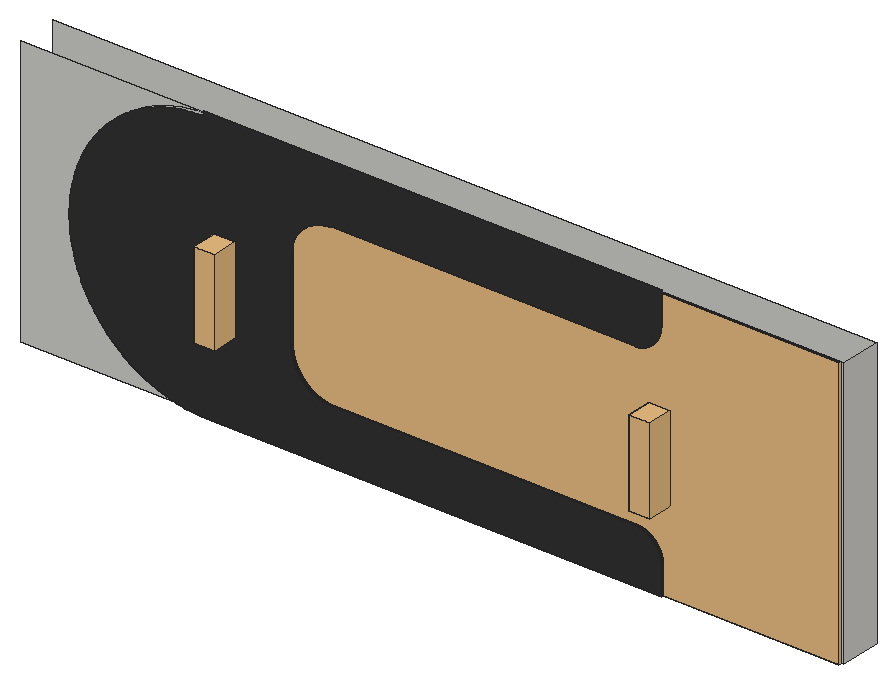
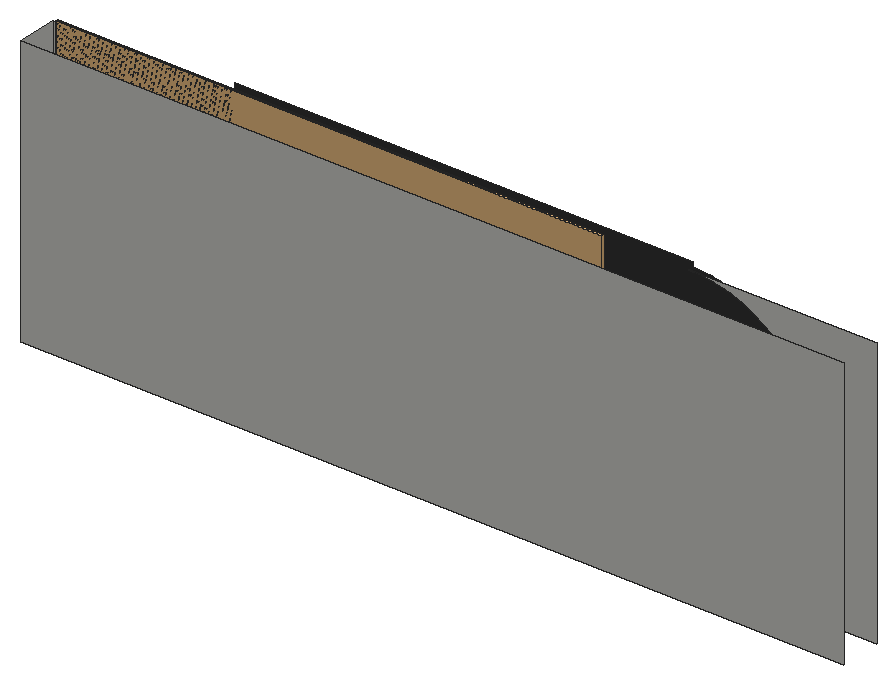
# SketchUp Ruby script. Lengths in inches.
U = 1.inch
M = Sketchup.active_model
def pt(a) = Geom::Point3d.new(a.map { |v| v * U })
def face(e, loops, mat)
  f = e.add_face(loops[0].map { |a| pt(a) })
  loops[1..].each { |l| e.add_face(l.map { |a| pt(a) }).erase! }
  f.material = f.back_material = mat if mat
  f
end
# faces: each face lists its corners as indices into pts; further lists are holes
def faces(e, pts, list, mat = nil) = list.each { |f| face(e, (f[0].is_a?(Array) ? f : [f]).map { |l| l.map { |i| pts[i] } }, mat) }
# xy, xz, yz: faces in a plane at the given z, y or x. An outline is a flat list of corners, or four numbers for a rectangle; further outlines are holes
def ring(l) = l.size == 4 ? [[l[0], l[1]], [l[2], l[1]], [l[2], l[3]], [l[0], l[3]]] : l.each_slice(2).to_a
def flat(e, list, mat, &to3) = list.each { |f| face(e, (f[0].is_a?(Array) ? f : [f]).map { |l| ring(l).map { |u, v| to3.(u, v) } }, mat) }
def xy(e, z, list, mat = nil) = flat(e, list, mat) { |x, y| [x, y, z] }
def xz(e, y, list, mat = nil) = flat(e, list, mat) { |x, z| [x, y, z] }
def yz(e, x, list, mat = nil) = flat(e, list, mat) { |y, z| [x, y, z] }
def lines(e, pts, list) = list.each { |a, b| e.add_line(pt(pts[a]), pt(pts[b])) }
# prism: a flat outline (further loops are holes) pulled along v
def prism(e, loops, v, mat = nil)
  f = face(e, loops, mat); d = Geom::Vector3d.new(v.map { |x| x * U })
  f.pushpull(f.normal.samedirection?(d) ? d.length : -d.length)
end
def box(e, o, s, mat = nil) = prism(e, [[o, [o[0] + s[0], o[1], o[2]], [o[0] + s[0], o[1] + s[1], o[2]], [o[0], o[1] + s[1], o[2]]]], [0, 0, s[2]], mat)
def at(x, y, z, deg = 0) = Geom::Transformation.translation(pt([x, y, z])) * Geom::Transformation.rotation(ORIGIN, Z_AXIS, deg.degrees)
def axes(o, x, y, z) = Geom::Transformation.new([*x, 0, *y, 0, *z, 0, *pt(o).to_a, 1])
def part(name) = M.definitions.add(name)
# library, detail: a bought-in or finely detailed component or shape, given as its bounding box
def library(name, o, s) = part(name).tap { |d| box(d.entities, o, s) }
def detail(e, o, s) = box(e.add_group.entities, o, s)
def put(e, d, t, mat = nil) = e.add_instance(d, t).tap { |i| i.material = mat if mat }
def group(e, t, mat = nil) = e.add_group.tap { |g| g.transformation = t; g.material = mat if mat }.entities
root = M.entities
M.materials.add("[Granite Dark Gray]").color = [51, 50, 50]
M.materials.add("[Stone Sandstone Ashlar Light]").color = [206, 205, 201]
M.materials.add("[Wood Cherry Original]").color = [118, 74, 44]
c1 = library("WALL LIGHT 69",[4.19,4.05,-9.63],[4.61,5.7,18.83])
c2 = library("Group\#156",[0,-0.5,0],[119.5,0.5,59])
xy(root,6,[[520.54,53,521,54]],"[Granite Dark Gray]")
xy(root,18,[[548.84,53,549,54],[549,53,615,54],[615,53,615.12,54],[615.12,53,615.24,54]],"[Granite Dark Gray]")
xy(root,18.01,[[548.53,53,548.6875,54]],"[Granite Dark Gray]")
xz(root,53,[[520.54,6,621,6,621,12.24,620.99,12.35,620.96,12.71,620.94,12.82,620.93,12.9375,620.91,13.05,620.88,13.17,620.86,13.29,620.83,13.4,620.81,13.51,620.77,13.63,620.71,13.85,620.67,13.97,620.63,14.08,620.59,14.1875,620.54,14.3,620.5,14.4,620.4,14.62,620.35,14.72,620.29,14.83,620.23,14.93,620.18,15.03,620.12,15.13,620.05,15.23,619.99,15.33,619.85,15.53,619.71,15.71,619.64,15.81,619.5625,15.9,619.49,15.99,619.41,16.07,619.33,16.16,619.24,16.24,619.16,16.33,619.07,16.41,618.99,16.49,618.9,16.5625,618.81,16.64,618.71,16.71,618.53,16.85,618.33,16.99,618.23,17.05,618.13,17.12,618.03,17.18,617.93,17.23,617.83,17.29,617.72,17.35,617.62,17.4,617.4,17.5,617.3,17.54,617.1875,17.59,617.08,17.63,616.97,17.67,616.85,17.71,616.63,17.77,616.51,17.81,616.4,17.83,616.29,17.86,616.17,17.88,616.05,17.91,615.9375,17.93,615.82,17.94,615.71,17.96,615.35,17.99,615.24,18,548.84,18,548.6875,18.01,548.53,18.01,548.37,18.02,548.22,18.03,547.9,18.07,547.75,18.09,547.59,18.11,547.4375,18.14,547.28,18.17,546.98,18.23,546.82,18.27,546.37,18.39,545.92,18.54,545.77,18.6,545.63,18.66,545.48,18.72,545.2,18.84,545.05,18.91,544.77,19.05,544.64,19.13,544.36,19.29,544.1,19.45,543.71,19.72,543.58,19.8125,543.46,19.91,543.34,20.01,543.21,20.11,543.1,20.21,542.98,20.3125,542.86,20.42,542.42,20.86,542.3125,20.98,542.21,21.1,542.11,21.21,542.01,21.34,541.91,21.46,541.8125,21.58,541.72,21.71,541.45,22.1,541.29,22.36,541.13,22.64,541.05,22.77,540.91,23.05,540.84,23.2,540.72,23.48,540.66,23.63,540.6,23.77,540.54,23.92,540.39,24.37,540.27,24.82,540.23,24.98,540.17,25.28,540.14,25.4375,540.11,25.59,540.09,25.75,540.07,25.9,540.03,26.22,540.02,26.37,540.01,26.53,540.01,26.6875,540,26.84,540,44.16,540.01,44.3125,540.01,44.47,540.02,44.63,540.03,44.78,540.07,45.1,540.09,45.25,540.11,45.41,540.14,45.5625,540.17,45.72,540.23,46.02,540.27,46.18,540.39,46.63,540.54,47.08,540.6,47.23,540.66,47.37,540.72,47.52,540.84,47.8,540.91,47.95,541.05,48.23,541.13,48.36,541.29,48.64,541.45,48.9,541.72,49.29,541.8125,49.42,541.91,49.54,542.01,49.66,542.11,49.79,542.21,49.9,542.3125,50.02,542.42,50.14,542.86,50.58,542.98,50.6875,543.1,50.79,543.21,50.89,543.34,50.99,543.46,51.09,543.58,51.1875,543.71,51.28,544.1,51.55,544.36,51.71,544.64,51.87,544.77,51.95,545.05,52.09,545.2,52.16,545.48,52.28,545.63,52.34,545.77,52.4,545.92,52.46,546.37,52.61,546.82,52.73,546.98,52.77,547.28,52.83,547.4375,52.86,547.59,52.89,547.75,52.91,547.9,52.93,548.22,52.97,548.37,52.98,548.53,52.99,548.6875,52.99,548.84,53,615.24,53,615.35,53.01,615.71,53.04,615.82,53.06,615.9375,53.07,616.05,53.09,616.17,53.12,616.29,53.14,616.4,53.17,616.51,53.19,616.63,53.23,616.85,53.29,616.97,53.33,617.08,53.37,617.1875,53.41,617.3,53.46,617.4,53.5,617.62,53.6,617.72,53.65,617.83,53.71,617.93,53.77,618.03,53.82,618.13,53.88,618.23,53.95,618.33,54.01,618.53,54.15,618.71,54.29,618.81,54.36,618.9,54.4375,618.99,54.51,619.07,54.59,619.16,54.67,619.24,54.76,619.33,54.84,619.41,54.93,619.49,55.01,619.5625,55.1,619.64,55.19,619.71,55.29,619.85,55.47,619.99,55.67,620.05,55.77,620.12,55.87,620.18,55.97,620.23,56.07,620.29,56.17,620.35,56.28,620.4,56.38,620.5,56.6,620.54,56.7,620.59,56.8125,620.63,56.92,620.67,57.03,620.71,57.15,620.77,57.37,620.81,57.49,620.83,57.6,620.86,57.71,620.88,57.83,620.91,57.95,620.93,58.0625,620.94,58.18,620.96,58.29,620.99,58.65,621,58.76,621,66,521,66,521,65,520.54,65,520.07,64.99,519.61,64.97,518.69,64.91,518.22,64.87,517.3,64.77,516.84,64.71,516.39,64.64,515.93,64.5625,515.47,64.48,515.02,64.39,514.56,64.29,513.66,64.07,513.22,63.95,512.77,63.83,512.33,63.7,511.88,63.56,511.44,63.41,511.01,63.26,510.57,63.1,510.14,62.93,509.28,62.57,508.86,62.39,508.02,61.99,507.2,61.57,506.79,61.35,506.38,61.125,505.98,60.89,505.59,60.65,505.19,60.41,504.8,60.16,504.04,59.64,503.66,59.37,502.92,58.81,502.2,58.23,501.84,57.93,501.49,57.63,501.15,57.32,500.47,56.68,500.14,56.36,499.82,56.03,499.18,55.35,498.87,55.01,498.57,54.66,498.27,54.3,497.69,53.58,497.13,52.84,496.86,52.46,496.34,51.7,496.09,51.31,495.85,50.91,495.61,50.52,495.375,50.12,495.15,49.71,494.93,49.3,494.51,48.48,494.11,47.64,493.93,47.22,493.57,46.36,493.4,45.93,493.24,45.49,493.09,45.06,492.94,44.62,492.8,44.17,492.67,43.73,492.55,43.28,492.43,42.84,492.21,41.94,492.11,41.48,492.02,41.03,491.9375,40.57,491.86,40.11,491.79,39.66,491.73,39.2,491.63,38.28,491.59,37.81,491.53,36.89,491.51,36.43,491.5,35.96,491.5,35.04,491.51,34.57,491.53,34.11,491.59,33.19,491.63,32.72,491.73,31.8,491.79,31.34,491.86,30.89,491.9375,30.43,492.02,29.97,492.11,29.52,492.21,29.06,492.43,28.16,492.55,27.72,492.67,27.27,492.8,26.83,492.94,26.38,493.09,25.94,493.24,25.51,493.4,25.07,493.57,24.64,493.93,23.78,494.11,23.36,494.51,22.52,494.93,21.7,495.15,21.29,495.375,20.88,495.61,20.48,495.85,20.09,496.09,19.69,496.34,19.3,496.86,18.54,497.13,18.16,497.69,17.42,498.27,16.7,498.57,16.34,498.87,15.99,499.18,15.65,499.82,14.97,500.14,14.64,500.47,14.32,501.15,13.68,501.49,13.37,501.84,13.07,502.2,12.77,502.92,12.19,503.66,11.63,504.04,11.36,504.8,10.84,505.19,10.59,505.59,10.35,505.98,10.11,506.38,9.875,506.79,9.65,507.2,9.43,508.02,9.01,508.86,8.61,509.28,8.43,510.14,8.07,510.57,7.9,511.01,7.74,511.44,7.59,511.88,7.44,512.33,7.3,512.77,7.17,513.22,7.05,513.66,6.93,514.56,6.71,515.02,6.61,515.47,6.52,515.93,6.4375,516.39,6.36,516.84,6.29,517.3,6.23,518.22,6.13,518.69,6.09,519.61,6.03,520.07,6.01]],"[Granite Dark Gray]")
xz(root,54,[[480,6,521,6,520.54,6,520.07,6.01,519.61,6.03,518.69,6.09,518.22,6.13,517.3,6.23,516.84,6.29,516.39,6.36,515.93,6.4375,515.47,6.52,515.02,6.61,514.56,6.71,513.66,6.93,513.22,7.05,512.77,7.17,512.33,7.3,511.88,7.44,511.44,7.59,511.01,7.74,510.57,7.9,510.14,8.07,509.28,8.43,508.86,8.61,508.02,9.01,507.2,9.43,506.79,9.65,506.38,9.875,505.98,10.11,505.59,10.35,505.19,10.59,504.8,10.84,504.04,11.36,503.66,11.63,502.92,12.19,502.2,12.77,501.84,13.07,501.49,13.37,501.15,13.68,500.47,14.32,500.14,14.64,499.82,14.97,499.18,15.65,498.87,15.99,498.57,16.34,498.27,16.7,497.69,17.42,497.13,18.16,496.86,18.54,496.34,19.3,496.09,19.69,495.85,20.09,495.61,20.48,495.375,20.88,495.15,21.29,494.93,21.7,494.51,22.52,494.11,23.36,493.93,23.78,493.57,24.64,493.4,25.07,493.24,25.51,493.09,25.94,492.94,26.38,492.8,26.83,492.67,27.27,492.55,27.72,492.43,28.16,492.21,29.06,492.11,29.52,492.02,29.97,491.9375,30.43,491.86,30.89,491.79,31.34,491.73,31.8,491.63,32.72,491.59,33.19,491.53,34.11,491.51,34.57,491.5,35.04,491.5,35.96,491.51,36.43,491.53,36.89,491.59,37.81,491.63,38.28,491.73,39.2,491.79,39.66,491.86,40.11,491.9375,40.57,492.02,41.03,492.11,41.48,492.21,41.94,492.43,42.84,492.55,43.28,492.67,43.73,492.8,44.17,492.94,44.62,493.09,45.06,493.24,45.49,493.4,45.93,493.57,46.36,493.93,47.22,494.11,47.64,494.51,48.48,494.93,49.3,495.15,49.71,495.375,50.12,495.61,50.52,495.85,50.91,496.09,51.31,496.34,51.7,496.86,52.46,497.13,52.84,497.69,53.58,498.27,54.3,498.57,54.66,498.87,55.01,499.18,55.35,499.82,56.03,500.14,56.36,500.47,56.68,501.15,57.32,501.49,57.63,501.84,57.93,502.2,58.23,502.92,58.81,503.66,59.37,504.04,59.64,504.8,60.16,505.19,60.41,505.59,60.65,505.98,60.89,506.38,61.125,506.79,61.35,507.2,61.57,508.02,61.99,508.86,62.39,509.28,62.57,510.14,62.93,510.57,63.1,511.01,63.26,511.44,63.41,511.88,63.56,512.33,63.7,512.77,63.83,513.22,63.95,513.66,64.07,514.56,64.29,515.02,64.39,515.47,64.48,515.93,64.5625,516.39,64.64,516.84,64.71,517.3,64.77,518.22,64.87,518.69,64.91,519.61,64.97,520.07,64.99,520.54,65,521,65,480,65],[621,6,660,6,660,65,621,65,621,58.76,620.99,58.65,620.96,58.29,620.94,58.18,620.93,58.0625,620.91,57.95,620.88,57.83,620.86,57.71,620.83,57.6,620.81,57.49,620.77,57.37,620.71,57.15,620.67,57.03,620.63,56.92,620.59,56.8125,620.54,56.7,620.5,56.6,620.4,56.38,620.35,56.28,620.29,56.17,620.23,56.07,620.18,55.97,620.12,55.87,620.05,55.77,619.99,55.67,619.85,55.47,619.71,55.29,619.64,55.19,619.5625,55.1,619.49,55.01,619.41,54.93,619.33,54.84,619.24,54.76,619.16,54.67,619.07,54.59,618.99,54.51,618.9,54.4375,618.81,54.36,618.71,54.29,618.53,54.15,618.33,54.01,618.23,53.95,618.13,53.88,618.03,53.82,617.93,53.77,617.83,53.71,617.72,53.65,617.62,53.6,617.4,53.5,617.3,53.46,617.1875,53.41,617.08,53.37,616.97,53.33,616.85,53.29,616.63,53.23,616.51,53.19,616.4,53.17,616.29,53.14,616.17,53.12,616.05,53.09,615.9375,53.07,615.82,53.06,615.71,53.04,615.35,53.01,615.24,53,548.84,53,548.6875,52.99,548.53,52.99,548.37,52.98,548.22,52.97,547.9,52.93,547.75,52.91,547.59,52.89,547.4375,52.86,547.28,52.83,546.98,52.77,546.82,52.73,546.37,52.61,545.92,52.46,545.77,52.4,545.63,52.34,545.48,52.28,545.2,52.16,545.05,52.09,544.77,51.95,544.64,51.87,544.36,51.71,544.1,51.55,543.71,51.28,543.58,51.1875,543.46,51.09,543.34,50.99,543.21,50.89,543.1,50.79,542.98,50.6875,542.86,50.58,542.42,50.14,542.3125,50.02,542.21,49.9,542.11,49.79,542.01,49.66,541.91,49.54,541.8125,49.42,541.72,49.29,541.45,48.9,541.29,48.64,541.13,48.36,541.05,48.23,540.91,47.95,540.84,47.8,540.72,47.52,540.66,47.37,540.6,47.23,540.54,47.08,540.39,46.63,540.27,46.18,540.23,46.02,540.17,45.72,540.14,45.5625,540.11,45.41,540.09,45.25,540.07,45.1,540.03,44.78,540.02,44.63,540.01,44.47,540.01,44.3125,540,44.16,540,26.84,540.01,26.6875,540.01,26.53,540.02,26.37,540.03,26.22,540.07,25.9,540.09,25.75,540.11,25.59,540.14,25.4375,540.17,25.28,540.23,24.98,540.27,24.82,540.39,24.37,540.54,23.92,540.6,23.77,540.66,23.63,540.72,23.48,540.84,23.2,540.91,23.05,541.05,22.77,541.13,22.64,541.29,22.36,541.45,22.1,541.72,21.71,541.8125,21.58,541.91,21.46,542.01,21.34,542.11,21.21,542.21,21.1,542.3125,20.98,542.42,20.86,542.86,20.42,542.98,20.3125,543.1,20.21,543.21,20.11,543.34,20.01,543.46,19.91,543.58,19.8125,543.71,19.72,544.1,19.45,544.36,19.29,544.64,19.13,544.77,19.05,545.05,18.91,545.2,18.84,545.48,18.72,545.63,18.66,545.77,18.6,545.92,18.54,546.37,18.39,546.82,18.27,546.98,18.23,547.28,18.17,547.4375,18.14,547.59,18.11,547.75,18.09,547.9,18.07,548.22,18.03,548.37,18.02,548.53,18.01,548.6875,18.01,548.84,18,615.24,18,615.35,17.99,615.71,17.96,615.82,17.94,615.9375,17.93,616.05,17.91,616.17,17.88,616.29,17.86,616.4,17.83,616.51,17.81,616.63,17.77,616.85,17.71,616.97,17.67,617.08,17.63,617.1875,17.59,617.3,17.54,617.4,17.5,617.62,17.4,617.72,17.35,617.83,17.29,617.93,17.23,618.03,17.18,618.13,17.12,618.23,17.05,618.33,16.99,618.53,16.85,618.71,16.71,618.81,16.64,618.9,16.5625,618.99,16.49,619.07,16.41,619.16,16.33,619.24,16.24,619.33,16.16,619.41,16.07,619.49,15.99,619.5625,15.9,619.64,15.81,619.71,15.71,619.85,15.53,619.99,15.33,620.05,15.23,620.12,15.13,620.18,15.03,620.23,14.93,620.29,14.83,620.35,14.72,620.4,14.62,620.5,14.4,620.54,14.3,620.59,14.1875,620.63,14.08,620.67,13.97,620.71,13.85,620.77,13.63,620.81,13.51,620.83,13.4,620.86,13.29,620.88,13.17,620.91,13.05,620.93,12.9375,620.94,12.82,620.96,12.71,620.99,12.35,621,12.24]],"[Stone Sandstone Ashlar Light]")
xz(root,63,[[480,6,660,65]],"[Stone Sandstone Ashlar Light]")
yz(root,540,[[53,26.84,54,27],[53,27,54,44]],"[Granite Dark Gray]")
yz(root,540.01,[[53,26.53,54,26.6875]],"[Granite Dark Gray]")
yz(root,621,[[53,6,54,12],[53,12,54,12.12],[53,12.12,54,12.24]],"[Granite Dark Gray]")
yz(root,660,[[54,6,63,65]],"[Stone Sandstone Ashlar Light]")
p = [[519.15,54,6.06],[519.61,54,6.03],[519.61,53,6.03],[519.15,53,6.06],[520.07,54,6.01],[520.07,53,6.01],
  [520.54,54,6],[520.54,53,6],[517.76,54,6.18],[518.22,54,6.13],[518.22,53,6.13],[517.76,53,6.18],
  [518.69,54,6.09],[518.69,53,6.09],[516.84,54,6.29],[517.3,54,6.23],[517.3,53,6.23],[516.84,53,6.29],
  [516.39,54,6.36],[516.39,53,6.36],[515.47,54,6.52],[515.93,54,6.4375],[515.93,53,6.4375],[515.47,53,6.52],
  [515.02,54,6.61],[515.02,53,6.61],[514.56,54,6.71],[514.56,53,6.71],[514.11,54,6.82],[514.11,53,6.82],
  [513.66,54,6.93],[513.66,53,6.93],[513.22,54,7.05],[513.22,53,7.05],[512.77,54,7.17],[512.77,53,7.17],
  [512.33,54,7.3],[512.33,53,7.3],[511.88,54,7.44],[511.88,53,7.44],[511.44,54,7.59],[511.44,53,7.59],
  [511.01,54,7.74],[511.01,53,7.74],[510.57,54,7.9],[510.57,53,7.9],[510.14,54,8.07],[510.14,53,8.07],
  [509.71,54,8.25],[509.71,53,8.25],[509.28,54,8.43],[509.28,53,8.43],[508.86,54,8.61],[508.86,53,8.61],
  [508.44,54,8.81],[508.44,53,8.81],[508.02,54,9.01],[508.02,53,9.01],[507.61,54,9.22],[507.61,53,9.22],
  [507.2,54,9.43],[507.2,53,9.43],[506.79,54,9.65],[506.79,53,9.65],[506.38,54,9.875],[506.38,53,9.875],
  [505.98,54,10.11],[505.98,53,10.11],[505.59,54,10.35],[505.59,53,10.35],[505.19,54,10.59],[505.19,53,10.59],
  [504.8,54,10.84],[504.8,53,10.84],[504.42,54,11.1],[504.42,53,11.1],[504.04,54,11.36],[504.04,53,11.36],
  [503.66,54,11.63],[503.66,53,11.63],[503.29,54,11.91],[503.29,53,11.91],[502.92,54,12.19],[502.92,53,12.19],
  [502.56,54,12.48],[502.56,53,12.48],[621,54,12.24],[620.99,54,12.35],[620.99,53,12.35],[621,53,12.24],
  [620.98,54,12.47],[620.98,53,12.47],[502.2,54,12.77],[502.2,53,12.77],[620.97,54,12.59],[620.97,53,12.59],
  [620.96,54,12.71],[620.96,53,12.71],[620.94,54,12.82],[620.94,53,12.82],[501.84,54,13.07],[501.84,53,13.07],
  [620.93,54,12.9375],[620.93,53,12.9375],[620.91,54,13.05],[620.91,53,13.05],[501.49,54,13.37],[501.49,53,13.37],
  [620.88,54,13.17],[620.88,53,13.17],[620.86,54,13.29],[620.86,53,13.29],[620.83,54,13.4],[620.83,53,13.4],
  [620.81,54,13.51],[620.81,53,13.51],[620.77,54,13.63],[620.77,53,13.63],[620.74,54,13.74],[620.74,53,13.74],
  [620.71,54,13.85],[620.71,53,13.85],[620.67,54,13.97],[620.67,53,13.97],[620.63,54,14.08],[620.63,53,14.08],
  [620.59,54,14.1875],[620.59,53,14.1875],[620.54,54,14.3],[620.54,53,14.3],[620.5,54,14.4],[620.5,53,14.4],
  [620.45,54,14.51],[620.45,53,14.51],[620.4,54,14.62],[620.4,53,14.62],[620.35,54,14.72],[620.35,53,14.72],
  [620.29,54,14.83],[620.29,53,14.83],[620.23,54,14.93],[620.23,53,14.93],[620.18,54,15.03],[620.18,53,15.03],
  [620.12,54,15.13],[620.12,53,15.13],[620.05,54,15.23],[620.05,53,15.23],[619.99,54,15.33],[619.99,53,15.33],
  [619.92,54,15.43],[619.92,53,15.43],[619.85,54,15.53],[619.85,53,15.53],[619.78,54,15.62],[619.78,53,15.62],
  [619.71,54,15.71],[619.71,53,15.71],[619.64,54,15.81],[619.64,53,15.81],[619.5625,54,15.9],[619.5625,53,15.9],
  [619.49,54,15.99],[619.49,53,15.99],[619.41,54,16.07],[619.41,53,16.07],[619.33,54,16.16],[619.33,53,16.16],
  [619.24,54,16.24],[619.16,54,16.33],[619.16,53,16.33],[619.24,53,16.24],[619.07,54,16.41],[619.07,53,16.41],
  [618.99,54,16.49],[618.99,53,16.49],[618.9,54,16.5625],[618.9,53,16.5625],[618.81,54,16.64],[618.71,54,16.71],
  [618.71,53,16.71],[618.81,53,16.64],[618.62,54,16.78],[618.62,53,16.78],[618.53,54,16.85],[618.53,53,16.85],
  [618.43,54,16.92],[618.33,54,16.99],[618.33,53,16.99],[618.43,53,16.92],[618.23,54,17.05],[618.23,53,17.05],
  [618.13,54,17.12],[618.03,54,17.18],[618.03,53,17.18],[618.13,53,17.12],[617.93,54,17.23],[617.83,54,17.29],
  [617.83,53,17.29],[617.93,53,17.23],[617.72,54,17.35],[617.62,54,17.4],[617.62,53,17.4],[617.72,53,17.35],
  [617.51,54,17.45],[617.4,54,17.5],[617.4,53,17.5],[617.51,53,17.45],[617.3,54,17.54],[617.1875,54,17.59],
  [617.1875,53,17.59],[617.3,53,17.54],[617.08,54,17.63],[616.97,54,17.67],[616.97,53,17.67],[617.08,53,17.63],
  [616.74,54,17.74],[616.63,54,17.77],[616.63,53,17.77],[616.74,53,17.74],[616.85,54,17.71],[616.85,53,17.71],
  [616.4,54,17.83],[616.29,54,17.86],[616.29,53,17.86],[616.4,53,17.83],[616.51,54,17.81],[616.51,53,17.81],
  [615.82,54,17.94],[615.71,54,17.96],[615.71,53,17.96],[615.82,53,17.94],[615.9375,54,17.93],[615.9375,53,17.93],
  [616.05,54,17.91],[616.05,53,17.91],[616.17,54,17.88],[616.17,53,17.88],[548.06,54,18.05],[547.9,54,18.07],
  [547.9,53,18.07],[548.06,53,18.05],[548.22,54,18.03],[548.22,53,18.03],[548.37,54,18.02],[548.37,53,18.02],
  [548.53,54,18.01],[548.53,53,18.01],[548.84,54,18],[548.6875,54,18.01],[548.6875,53,18.01],[548.84,53,18],
  [615.35,54,17.99],[615.24,54,18],[615.24,53,18],[615.35,53,17.99],[615.47,54,17.98],[615.47,53,17.98],
  [615.59,54,17.97],[615.59,53,17.97],[547.4375,54,18.14],[547.28,54,18.17],[547.28,53,18.17],[547.4375,53,18.14],
  [547.59,54,18.11],[547.59,53,18.11],[547.75,54,18.09],[547.75,53,18.09],[546.98,54,18.23],[546.82,54,18.27],
  [546.82,53,18.27],[546.98,53,18.23],[547.13,54,18.2],[547.13,53,18.2],[546.52,54,18.35],[546.37,54,18.39],
  [546.37,53,18.39],[546.52,53,18.35],[546.67,54,18.31],[546.67,53,18.31],[546.22,54,18.44],[546.07,54,18.49],
  [546.07,53,18.49],[546.22,53,18.44],[545.92,54,18.54],[545.77,54,18.6],[545.77,53,18.6],[545.92,53,18.54],
  [545.63,54,18.66],[545.63,53,18.66],[545.48,54,18.72],[545.34,54,18.78],[545.34,53,18.78],[545.48,53,18.72],
  [545.2,54,18.84],[545.05,54,18.91],[545.05,53,18.91],[545.2,53,18.84],[544.91,54,18.98],[544.91,53,18.98],
  [544.77,54,19.05],[544.77,53,19.05],[544.64,54,19.13],[544.5,54,19.21],[544.5,53,19.21],[544.64,53,19.13],
  [544.36,54,19.29],[544.36,53,19.29],[544.23,54,19.37],[544.23,53,19.37],[544.1,54,19.45],[544.1,53,19.45],
  [543.97,54,19.54],[543.84,54,19.63],[543.84,53,19.63],[543.97,53,19.54],[543.71,54,19.72],[543.71,53,19.72],
  [543.58,54,19.8125],[543.58,53,19.8125],[543.46,54,19.91],[543.46,53,19.91],[543.34,54,20.01],[543.34,53,20.01],
  [543.21,54,20.11],[543.21,53,20.11],[543.1,54,20.21],[543.1,53,20.21],[542.98,54,20.3125],[542.98,53,20.3125],
  [542.86,54,20.42],[542.86,53,20.42],[542.75,54,20.53],[542.75,53,20.53],[542.64,54,20.64],[542.64,53,20.64],
  [542.53,54,20.75],[542.53,53,20.75],[542.42,54,20.86],[542.42,53,20.86],[542.3125,54,20.98],[542.3125,53,20.98],
  [542.21,54,21.1],[542.21,53,21.1],[542.11,54,21.21],[542.11,53,21.21],[542.01,54,21.34],[542.01,53,21.34],
  [541.91,54,21.46],[541.91,53,21.46],[541.8125,54,21.58],[541.8125,53,21.58],[541.72,54,21.71],[541.72,53,21.71],
  [541.63,54,21.84],[541.63,53,21.84],[541.54,54,21.97],[541.54,53,21.97],[541.45,54,22.1],[541.45,53,22.1],
  [541.37,54,22.23],[541.37,53,22.23],[541.29,54,22.36],[541.29,53,22.36],[541.21,54,22.5],[541.21,53,22.5],
  [541.13,54,22.64],[541.13,53,22.64],[541.05,54,22.77],[541.05,53,22.77],[540.98,54,22.91],[540.98,53,22.91],
  [540.91,54,23.05],[540.91,53,23.05],[540.84,54,23.2],[540.84,53,23.2],[540.78,54,23.34],[540.78,53,23.34],
  [540.72,54,23.48],[540.72,53,23.48],[540.66,54,23.63],[540.66,53,23.63],[540.6,54,23.77],[540.6,53,23.77],
  [540.54,54,23.92],[540.54,53,23.92],[540.49,54,24.07],[540.49,53,24.07],[540.44,54,24.22],[540.44,53,24.22],
  [540.39,54,24.37],[540.39,53,24.37],[540.35,54,24.52],[540.35,53,24.52],[540.31,54,24.67],[540.31,53,24.67],
  [540.27,54,24.82],[540.27,53,24.82],[540.23,54,24.98],[540.23,53,24.98],[540.2,54,25.13],[540.2,53,25.13],
  [540.17,54,25.28],[540.17,53,25.28],[540.14,54,25.4375],[540.14,53,25.4375],[540.11,54,25.59],[540.11,53,25.59],
  [540.09,54,25.75],[540.09,53,25.75],[540.07,54,25.9],[540.07,53,25.9],[540.05,54,26.06],[540.05,53,26.06],
  [540.03,54,26.22],[540.03,53,26.22],[540.02,54,26.37],[540.02,53,26.37],[540.01,54,26.53],[540.01,53,26.53],
  [540.01,54,26.6875],[540,54,26.84],[540,53,26.84],[540.01,53,26.6875]]
faces(root,p,[[0,1,2,3],[1,4,5,2],[4,6,7,5],[8,9,10,11],[9,12,13,10],[12,0,3,13],[14,15,16,17],[15,8,11,16],
  [18,14,17,19],[20,21,22,23],[21,18,19,22],[24,20,23,25],[26,24,25,27],[28,26,27,29],[30,28,29,31],[32,30,31,33],
  [34,32,33,35],[36,34,35,37],[38,36,37,39],[40,38,39,41],[42,40,41,43],[44,42,43,45],[46,44,45,47],[48,46,47,49],
  [50,48,49,51],[52,50,51,53],[54,52,53,55],[56,54,55,57],[58,56,57,59],[60,58,59,61],[62,60,61,63],[64,62,63,65],
  [66,64,65,67],[68,66,67,69],[70,68,69,71],[72,70,71,73],[74,72,73,75],[76,74,75,77],[78,76,77,79],[80,78,79,81],
  [82,80,81,83],[84,82,83,85],[86,87,88,89],[87,90,91,88],[92,84,85,93],[90,94,95,91],[94,96,97,95],[96,98,99,97],
  [100,92,93,101],[98,102,103,99],[102,104,105,103],[106,100,101,107],[104,108,109,105],[108,110,111,109],[110,112,113,111],[112,114,115,113],
  [114,116,117,115],[116,118,119,117],[118,120,121,119],[120,122,123,121],[122,124,125,123],[124,126,127,125],[126,128,129,127],[128,130,131,129],
  [130,132,133,131],[132,134,135,133],[134,136,137,135],[136,138,139,137],[138,140,141,139],[140,142,143,141],[142,144,145,143],[144,146,147,145],
  [146,148,149,147],[148,150,151,149],[150,152,153,151],[152,154,155,153],[154,156,157,155],[156,158,159,157],[158,160,161,159],[160,162,163,161],
  [162,164,165,163],[164,166,167,165],[168,169,170,171],[166,168,171,167],[169,172,173,170],[172,174,175,173],[174,176,177,175],[178,179,180,181],
  [176,178,181,177],[179,182,183,180],[182,184,185,183],[186,187,188,189],[184,186,189,185],[187,190,191,188],[192,193,194,195],[190,192,195,191],
  [196,197,198,199],[193,196,199,194],[200,201,202,203],[197,200,203,198],[204,205,206,207],[201,204,207,202],[208,209,210,211],[205,208,211,206],
  [212,213,214,215],[209,212,215,210],[216,217,218,219],[220,216,219,221],[213,220,221,214],[222,223,224,225],[226,222,225,227],[217,226,227,218],
  [228,229,230,231],[232,228,231,233],[234,232,233,235],[236,234,235,237],[223,236,237,224],[238,239,240,241],[242,238,241,243],[244,242,243,245],
  [246,244,245,247],[248,249,250,251],[252,253,254,255],[256,252,255,257],[258,256,257,259],[229,258,259,230],[260,261,262,263],[264,260,263,265],
  [266,264,265,267],[239,266,267,240],[268,269,270,271],[272,268,271,273],[261,272,273,262],[274,275,276,277],[278,274,277,279],[269,278,279,270],
  [280,281,282,283],[275,280,283,276],[284,285,286,287],[281,284,287,282],[285,288,289,286],[290,291,292,293],[288,290,293,289],[294,295,296,297],
  [291,294,297,292],[295,298,299,296],[298,300,301,299],[302,303,304,305],[300,302,305,301],[303,306,307,304],[306,308,309,307],[308,310,311,309],
  [312,313,314,315],[310,312,315,311],[313,316,317,314],[316,318,319,317],[318,320,321,319],[320,322,323,321],[322,324,325,323],[324,326,327,325],
  [326,328,329,327],[328,330,331,329],[330,332,333,331],[332,334,335,333],[334,336,337,335],[336,338,339,337],[338,340,341,339],[340,342,343,341],
  [342,344,345,343],[344,346,347,345],[346,348,349,347],[348,350,351,349],[350,352,353,351],[352,354,355,353],[354,356,357,355],[356,358,359,357],
  [358,360,361,359],[360,362,363,361],[362,364,365,363],[364,366,367,365],[366,368,369,367],[368,370,371,369],[370,372,373,371],[372,374,375,373],
  [374,376,377,375],[376,378,379,377],[378,380,381,379],[380,382,383,381],[382,384,385,383],[384,386,387,385],[386,388,389,387],[388,390,391,389],
  [390,392,393,391],[392,394,395,393],[394,396,397,395],[396,398,399,397],[398,400,401,399],[400,402,403,401],[402,404,405,403],[404,406,407,405],
  [406,408,409,407],[408,410,411,409],[410,412,413,411],[412,414,415,413],[414,416,417,415],[416,418,419,417],[420,421,422,423]],"[Granite Dark Gray]")
put(root,c1,at(519.01,43.25,33.5625))
put(root,c2,at(540,54,6),"[Wood Cherry Original]")
put(root,c1,at(613.7,44,33.5625))
